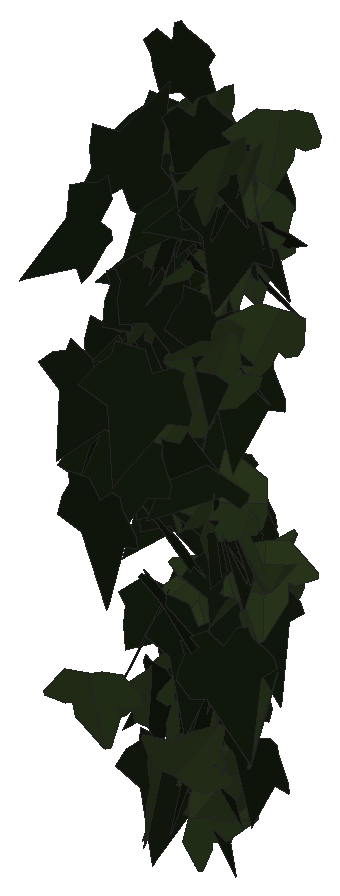
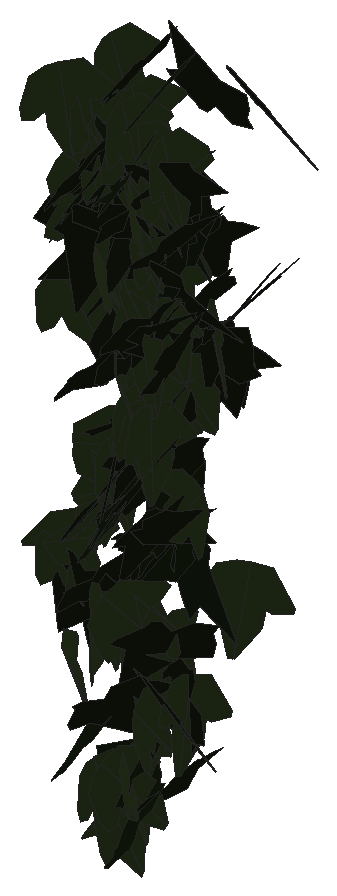
# SketchUp Ruby script. Lengths in inches.
U = 1.inch
M = Sketchup.active_model
def pt(a) = Geom::Point3d.new(a.map { |v| v * U })
def face(e, loops, mat)
  f = e.add_face(loops[0].map { |a| pt(a) })
  loops[1..].each { |l| e.add_face(l.map { |a| pt(a) }).erase! }
  f.material = f.back_material = mat if mat
  f
end
# faces: each face lists its corners as indices into pts; further lists are holes
def faces(e, pts, list, mat = nil) = list.each { |f| face(e, (f[0].is_a?(Array) ? f : [f]).map { |l| l.map { |i| pts[i] } }, mat) }
# xy, xz, yz: faces in a plane at the given z, y or x. An outline is a flat list of corners, or four numbers for a rectangle; further outlines are holes
def ring(l) = l.size == 4 ? [[l[0], l[1]], [l[2], l[1]], [l[2], l[3]], [l[0], l[3]]] : l.each_slice(2).to_a
def flat(e, list, mat, &to3) = list.each { |f| face(e, (f[0].is_a?(Array) ? f : [f]).map { |l| ring(l).map { |u, v| to3.(u, v) } }, mat) }
def xy(e, z, list, mat = nil) = flat(e, list, mat) { |x, y| [x, y, z] }
def xz(e, y, list, mat = nil) = flat(e, list, mat) { |x, z| [x, y, z] }
def yz(e, x, list, mat = nil) = flat(e, list, mat) { |y, z| [x, y, z] }
def lines(e, pts, list) = list.each { |a, b| e.add_line(pt(pts[a]), pt(pts[b])) }
# prism: a flat outline (further loops are holes) pulled along v
def prism(e, loops, v, mat = nil)
  f = face(e, loops, mat); d = Geom::Vector3d.new(v.map { |x| x * U })
  f.pushpull(f.normal.samedirection?(d) ? d.length : -d.length)
end
def box(e, o, s, mat = nil) = prism(e, [[o, [o[0] + s[0], o[1], o[2]], [o[0] + s[0], o[1] + s[1], o[2]], [o[0], o[1] + s[1], o[2]]]], [0, 0, s[2]], mat)
def at(x, y, z, deg = 0) = Geom::Transformation.translation(pt([x, y, z])) * Geom::Transformation.rotation(ORIGIN, Z_AXIS, deg.degrees)
def axes(o, x, y, z) = Geom::Transformation.new([*x, 0, *y, 0, *z, 0, *pt(o).to_a, 1])
def part(name) = M.definitions.add(name)
# library, detail: a bought-in or finely detailed component or shape, given as its bounding box
def library(name, o, s) = part(name).tap { |d| box(d.entities, o, s) }
def detail(e, o, s) = box(e.add_group.entities, o, s)
def put(e, d, t, mat = nil) = e.add_instance(d, t).tap { |i| i.material = mat if mat }
def group(e, t, mat = nil) = e.add_group.tap { |g| g.transformation = t; g.material = mat if mat }.entities
root = M.entities
M.materials.add("efeu1").color = [18, 25, 13]
M.materials.add("efeu2").color = [43, 57, 29]
c1 = part("ivyleaf_10")
p = [[0,0.5,-0.03],[-0.0625,2.02,-0.43],[-0.19,2.01,-0.46],[-0.54,1.05,-0.29],[-0.52,0.625,-0.18],[-0.83,0.76,-0.28],
  [-1.16,0.64,-0.33],[-1.15,0.33,-0.24],[-0.77,-0.39,0.02],[-0.3,-0.51,0.16],[0.04,-0.48,0.23],[-0.02,2.01,-0.4375],
  [-0.06,2.01,-0.43],[0.04,-0.49,0.23],[0.67,-0.49,0.14],[1.38,0.36,-0.2],[1.375,0.51,-0.24],[0.81,0.65,-0.19],
  [0.62,0.59,-0.15],[0.6,1.09,-0.28],[0.5,1.23,-0.31]]
faces(c1.entities,p,[[0,1,2,3,4,5,6,7,8,9,10],[11,12,0,13,14,15,16,17,18,19,20]],"efeu2")
c2 = part("ivyleaf_9")
p = [[1.54,2.16,1.25],[1.36,2.04,1.19],[-0.21,0.99,0.68],[-0.71,1.11,0.82],[-0.85,0.86,0.67],[-0.8,0.17,0.21],
  [-0.9,-0.01,0.1],[-0.67,-0.16,-0.02],[-0.08,-0.08,-0.05],[-0.03,-0.6,-0.4],[0.65,-0.88,-0.66],[0.83,-0.6,-0.49],
  [1.29,-0.42,-0.43],[1.8125,-0.07,-0.26],[1.21,0.44,0.15]]
faces(c2.entities,p,[[0,1,2,3,4,5,6,7,8,9,10,11,12,13,14]],"efeu1")
put(root,c1,axes([18.49,222.43,229.99],[0.23002,-0.33057,-0.29633],[-0.15826,0.25076,-0.40258],[0.41478,0.279,0.01073]))
put(root,c1,axes([18.22,223.25,227.8],[-0.37574,0.15973,-0.28863],[0.24252,-0.1628,-0.40581],[-0.22361,-0.44495,0.04487]))
put(root,c1,axes([18.43,222.98,224.79],[-0.0906,-0.46509,-0.15963],[0.04334,0.15413,-0.47367],[0.48981,-0.09967,0.01238]))
put(root,c2,axes([18.42,223.59,229.8],[-0.11921,-0.27208,0.4022],[-0.12254,-0.38388,-0.29601],[0.46986,-0.16914,0.02485]))
put(root,c1,axes([18.51,223.32,232.72],[0.01604,-0.49871,0.03217],[0.00614,-0.03199,-0.49894],[0.4997,0.0164,0.0051]))
put(root,c2,axes([18.41,223.64,231.55],[-0.15985,-0.43972,0.17633],[-0.02074,-0.17942,-0.46624],[0.47331,-0.15637,0.03912]))
put(root,c2,axes([18.82,223.33,230.9],[-0.44717,0.10536,0.19733],[-0.19143,0.04795,-0.45941],[-0.11573,-0.48641,-0.00254]))
put(root,c2,axes([18.55,223.72,227.49],[-0.316,-0.3588,0.14632],[-0.04704,-0.1519,-0.47404],[0.38462,-0.31335,0.06225]))
put(root,c2,axes([18.72,223.49,225.0625],[-0.4789,0.12444,-0.0719],[0.07015,-0.01592,-0.4948],[-0.12544,-0.484,-0.00221]))
put(root,c2,axes([18.56,223.48,232.52],[-0.39863,-0.28258,-0.10604],[0.08305,0.06619,-0.48859],[0.29017,-0.40715,-0.00584]))
put(root,c1,axes([18.67,223.45,228.82],[-0.0673,-0.49025,-0.07159],[0.02179,0.06925,-0.4947],[0.49497,-0.0697,0.01205]))
put(root,c1,axes([18.71,223.16,232.33],[-0.07169,-0.46603,0.16637],[-0.02755,-0.16409,-0.4715],[0.49407,-0.07677,-0.00215]))
put(root,c2,axes([18.45,222.9,230.46],[0.08987,-0.48242,-0.09591],[-0.01598,0.09459,-0.49071],[0.4916,0.09126,0.00159]))
put(root,c2,axes([18.42,223.4,225.875],[0.00253,-0.37791,-0.32737],[0.11638,0.31883,-0.36715],[0.48626,-0.07435,0.08958]))
put(root,c2,axes([18.44,222.44,229.3125],[-0.24213,0.0676,0.43221],[0.40007,-0.16562,0.25003],[0.17697,0.4669,0.02611]))
put(root,c2,axes([18.86,223.4,229.93],[-0.33647,-0.18993,0.31735],[-0.2156,-0.24787,-0.37693],[0.30051,-0.39049,0.08491]))
put(root,c1,axes([18.72,222.76,229.12],[-0.09175,-0.40686,0.27576],[0.04283,-0.28607,-0.40783],[0.48964,-0.05122,0.08734]))
put(root,c1,axes([19,223.41,230.66],[0.24717,0.01492,-0.43438],[-0.43424,-0.01272,-0.24753],[-0.01844,0.49962,0.00667]))
put(root,c1,axes([18.77,223.36,231.46],[0.0213,-0.48092,0.13513],[-0.01137,-0.13569,-0.4811],[0.49942,0.01742,-0.01671]))
put(root,c2,axes([18.54,223.41,227.57],[0.11099,-0.41936,-0.24864],[-0.03846,0.24667,-0.43321],[0.48601,0.11529,0.0225]))
put(root,c1,axes([18.71,223.19,230.1],[0.00725,-0.44774,0.22243],[0.07343,-0.21909,-0.44341],[0.49453,0.0391,0.06258]))
put(root,c2,axes([18.82,221.67,229.08],[-0.02563,0.08745,-0.49162],[-0.30019,0.39069,0.08515],[0.39904,0.29952,0.03248]))
put(root,c2,axes([18.52,223.41,233.75],[0.28205,-0.39313,-0.12607],[-0.02753,0.13444,-0.4808],[0.41194,0.27816,0.05419]))
put(root,c1,axes([18.81,222.95,231.91],[0.01487,-0.49894,-0.02902],[-0.00396,0.02891,-0.49915],[0.49976,0.01507,-0.00309]))
put(root,c2,axes([18.625,223.22,223.5],[-0.06473,-0.47171,0.15265],[0.02959,-0.15735,-0.47367],[0.49491,-0.05229,0.04829]))
put(root,c1,axes([18.76,222.76,231.3],[0.11483,-0.39119,-0.28946],[0.0705,0.30764,-0.3878],[0.4815,0.04824,0.12581]))
put(root,c2,axes([18.42,223.23,231.15],[0.14483,-0.22385,0.42298],[0.26952,-0.32703,-0.26535],[0.39545,0.30487,0.02593]))
put(root,c2,axes([18.68,221.58,229.74],[-0.11819,-0.39915,0.27696],[0.02609,-0.28984,-0.40658],[0.48513,-0.08165,0.08934]))
put(root,c2,axes([18.4,223.13,231.45],[0.17859,-0.27091,0.38041],[0.314,-0.23182,-0.31251],[0.3457,0.35052,0.08733]))
put(root,c1,axes([18.72,223.54,224.57],[0.11366,-0.35039,0.3381],[0.15787,-0.30191,-0.36596],[0.46061,0.18994,0.042]))
put(root,c1,axes([18.86,221.34,225.57],[-0.46112,-0.19068,-0.03179],[0.0291,0.01282,-0.49899],[0.19111,-0.46203,-0.00073]))
put(root,c1,axes([19.03,223.7,226.125],[-0.19329,-0.28552,0.36211],[-0.16913,-0.32138,-0.34368],[0.429,-0.25534,0.02766]))
put(root,c1,axes([18.7,222.99,230.05],[-0.40483,0.16773,-0.24078],[0.20233,-0.13761,-0.43604],[-0.21254,-0.45048,0.04355]))
put(root,c2,axes([18.71,223.46,230.34],[-0.05512,-0.47784,-0.1365],[0.0033,0.13698,-0.48086],[0.49694,-0.05391,-0.01195]))
put(root,c2,axes([18.47,222.98,224.71],[0.0622,-0.02561,-0.49545],[0.48938,0.08517,0.05704],[0.08147,-0.49203,0.03566]))
put(root,c2,axes([18.66,223.59,228.18],[0.18627,-0.46146,-0.04853],[-0.01392,0.04671,-0.49762],[0.4638,0.18673,0.00455]))
put(root,c1,axes([19.11,223.12,229.8125],[-0.42756,0.04442,0.25538],[-0.25395,0.02698,-0.42986],[-0.05197,-0.49729,-0.00051]))
put(root,c1,axes([18.93,223.43,232],[0.17479,-0.46471,-0.05906],[-0.01428,0.05773,-0.49645],[0.46824,0.17524,0.00691]))
put(root,c1,axes([18.96,222.5,230.7],[0.07805,-0.4605,-0.17847],[-0.01785,0.17794,-0.46693],[0.49355,0.07925,0.01134]))
put(root,c1,axes([18.97,223.13,228.67],[-0.21243,-0.4516,-0.03047],[0.00717,0.0303,-0.49903],[0.45257,-0.21246,-0.00639]))
put(root,c2,axes([19.03,222.75,231.67],[-0.39202,0.19463,-0.24175],[0.21966,-0.10113,-0.43763],[-0.21925,-0.44932,-0.00621]))
put(root,c1,axes([19,223.33,232.72],[-0.23758,-0.43928,0.02424],[-0.00273,-0.02608,-0.49931],[0.43994,-0.23738,0.00999]))
put(root,c2,axes([19.22,220.96,232.51],[-0.4655,0.1808,0.0249],[-0.02444,0.00584,-0.49937],[-0.18086,-0.46613,0.00341]))
put(root,c2,axes([18.87,223.66,231.97],[-0.11651,-0.46381,0.14595],[-0.0226,-0.14475,-0.47805],[0.48571,-0.118,0.01277]))
put(root,c1,axes([19.09,223.67,223.67],[-0.09524,-0.37066,0.32177],[-0.09347,-0.30808,-0.38256],[0.48187,-0.13302,-0.01061]))
put(root,c1,axes([19.03,223.07,230.37],[0.24768,-0.41489,-0.12854],[-0.04106,0.12494,-0.48239],[0.4324,0.24951,0.02782]))
put(root,c1,axes([19.01,223.45,223.72],[0.15733,-0.4744,0.01374],[0.00443,-0.01301,-0.49981],[0.47458,0.15739,0.00011]))
put(root,c2,axes([19.07,223.08,232.2],[-0.31124,-0.35892,0.15592],[-0.04886,-0.16203,-0.47049],[0.38826,-0.3081,0.06579]))
put(root,c1,axes([18.79,223.43,225.97],[0.4352,0.07159,0.23553],[0.23055,0.04915,-0.44094],[-0.08629,0.4924,0.00977]))
put(root,c1,axes([19.09,223.42,233.07],[-0.02939,-0.49624,0.05371],[0.01107,-0.05443,-0.4969],[0.49901,-0.02802,0.01418]))
put(root,c1,axes([19.07,223.36,228.85],[0.01693,-0.4832,0.12739],[0.03041,-0.12623,-0.48285],[0.49879,0.02409,0.02511]))
put(root,c1,axes([19.08,223.22,230.73],[0.04276,-0.41979,0.26823],[0.02782,-0.26678,-0.42196],[0.49739,0.05101,0.00054]))
put(root,c2,axes([19.15,222.14,226.1875],[-0.32069,0.26618,-0.27623],[0.21379,-0.17493,-0.41677],[-0.31851,-0.38542,-0.00162]))
put(root,c2,axes([18.76,223.64,223.13],[0.22105,-0.39181,0.21821],[0.10401,-0.19186,-0.44986],[0.43625,0.24428,-0.00332]))
put(root,c2,axes([19.01,221.78,232.66],[-0.35569,0.20594,0.28473],[0.24474,-0.14554,0.411],[0.25216,0.43175,0.00273]))
put(root,c2,axes([18.79,222.91,227.1],[0.02735,-0.29699,0.40131],[0.24681,-0.34132,-0.26942],[0.43398,0.21283,0.12793]))
put(root,c1,axes([19.15,223.62,223.13],[0.03474,-0.46755,0.17377],[0.01106,-0.17342,-0.46883],[0.49867,0.03641,-0.00171]))
put(root,c2,axes([18.95,222.94,228.15],[-0.00928,-0.34731,-0.35957],[0.02564,0.35883,-0.34725],[0.49926,-0.02488,0.01115]))
put(root,c1,axes([19.09,223.02,224.97],[0.06128,-0.43269,0.24295],[0.1161,-0.2255,-0.43089],[0.48246,0.10922,0.07283]))
put(root,c2,axes([18.95,222.45,231.02],[0.14227,-0.44698,-0.1731],[-0.02881,0.17227,-0.4685],[0.47846,0.14329,0.02326]))
put(root,c1,axes([19.08,223.31,230.34],[-0.11055,-0.33535,0.354],[0.16948,-0.36678,-0.29453],[0.45723,0.05487,0.19476]))
put(root,c2,axes([19.16,223.75,224.8125],[-0.23283,-0.44165,0.02713],[-0.00804,-0.02643,-0.49924],[0.44241,-0.23291,0.0052]))
put(root,c1,axes([19.125,223.48,229.27],[0.33317,-0.31949,0.19216],[0.13828,-0.13343,-0.4616],[0.34623,0.36072,-0.00055]))
put(root,c2,axes([18.99,223.47,232.49],[0.2856,-0.4104,0.00221],[0.00128,-0.0018,-0.5],[0.4104,0.28561,0.00002]))
put(root,c1,axes([19.3,222.95,233.03],[-0.08013,-0.47509,0.13368],[0.00933,-0.13686,-0.48081],[0.49345,-0.07456,0.0308]))
put(root,c2,axes([19.09,223.04,228.64],[-0.14371,-0.3551,0.32133],[0.12506,-0.35167,-0.3327],[0.46229,-0.01525,0.18989]))
put(root,c2,axes([19.24,221.5625,228.95],[-0.36621,-0.30924,-0.14235],[0.1108,0.08942,-0.4793],[0.32189,-0.38259,0.00304]))
put(root,c1,axes([19.36,222.6,229.26],[-0.17602,-0.37038,0.28607],[-0.04394,-0.29121,-0.40406],[0.46593,-0.16739,0.06996]))
put(root,c2,axes([19.38,223.59,231.69],[-0.45532,-0.19539,-0.06712],[0.06362,0.02194,-0.49545],[0.19656,-0.45972,0.00488]))
put(root,c2,axes([18.95,223.52,223.67],[0.17403,-0.35204,0.30948],[0.17894,-0.25523,-0.39095],[0.43324,0.24683,0.03716]))
put(root,c1,axes([19.36,222.94,229.84],[0.00912,-0.41573,0.27764],[0.05426,-0.27522,-0.41389],[0.49696,0.03768,0.04009]))
put(root,c2,axes([19.12,223.72,228.09],[0.14057,-0.16887,-0.44914],[0.40301,-0.21246,0.20602],[-0.26043,-0.41993,0.07638]))
put(root,c1,axes([19.34,223.56,231.03],[0.1772,-0.41935,0.20676],[0.0732,-0.1935,-0.45519],[0.46178,0.19159,-0.00718]))
put(root,c2,axes([19.1,222.69,226.16],[0.00637,-0.31139,0.39115],[0.22861,-0.34608,-0.27923],[0.44463,0.1824,0.13797]))
put(root,c2,axes([19.1,223.49,227.6],[0.2118,-0.42089,0.16732],[0.07928,-0.14741,-0.47115],[0.44593,0.22611,0.0043]))
put(root,c1,axes([19.3,222.93,223.15],[0.07077,-0.21703,-0.44485],[0.18626,0.42802,-0.17919],[0.45858,-0.14035,0.14143]))
put(root,c2,axes([19.21,223.76,227.27],[0.01542,-0.37526,0.33006],[0.05245,-0.32718,-0.37444],[0.497,0.04617,0.02927]))
put(root,c1,axes([19.51,223.46,223.44],[-0.02066,-0.4994,0.01327],[-0.00139,-0.01322,-0.49982],[0.49957,-0.02069,-0.00084]))
put(root,c1,axes([19.5,223.375,226.08],[0.08402,-0.49207,-0.02848],[-0.00769,0.02758,-0.49918],[0.49283,0.08432,-0.00293]))
put(root,c2,axes([19.5625,223.09,228.41],[-0.32859,-0.31081,0.21314],[-0.03881,-0.25337,-0.4293],[0.37487,-0.29867,0.14238]))
put(root,c2,axes([19.3,223.08,232.28],[0.21048,-0.41575,-0.18125],[-0.04013,0.18197,-0.46398],[0.45176,0.20987,0.04324]))
put(root,c2,axes([19.16,223.33,229.82],[0.25074,-0.27453,0.33431],[0.23382,-0.23909,-0.3717],[0.36395,0.34274,0.00849]))
put(root,c2,axes([19.41,223.56,227.34],[-0.09365,-0.41897,0.2563],[0.05854,-0.26858,-0.41766],[0.48765,-0.04822,0.09936]))
put(root,c1,axes([19.77,222.96,231.41],[0.33072,-0.13862,-0.34844],[-0.31426,0.15104,-0.35837],[0.20461,0.45604,0.01278]))
put(root,c2,axes([19.48,223.61,226.39],[-0.13623,-0.47148,0.09566],[-0.00391,-0.09834,-0.49022],[0.48107,-0.13431,0.02311]))
put(root,c1,axes([19.62,223.03,227.84],[0.01891,-0.49879,0.02917],[0.00353,-0.02906,-0.49914],[0.49963,0.01908,0.00243]))
put(root,c2,axes([19.35,223.69,227.63],[0.11155,-0.46219,0.15472],[0.04348,-0.14865,-0.47541],[0.48545,0.11952,0.00703]))
put(root,c2,axes([19.26,223.31,231.28],[0.45873,-0.16514,0.11087],[0.10779,-0.02783,-0.48745],[0.16717,0.47112,0.01007]))
put(root,c2,axes([19.79,223.24,231.94],[-0.24308,-0.16784,0.40341],[-0.28493,-0.28909,-0.29196],[0.33125,-0.37183,0.0449]))
put(root,c2,axes([19.55,222.7,224.7],[-0.29017,0.05517,-0.40343],[0.37193,-0.16574,-0.29018],[-0.16575,-0.46849,0.05515]))
put(root,c2,axes([19.49,222.63,226.01],[0.00471,-0.48333,0.12796],[-0.00653,-0.12802,-0.48329],[0.49994,0.00288,-0.00752]))
put(root,c2,axes([19.85,222.85,232.43],[-0.41021,0.2599,-0.11906],[0.0992,-0.06588,-0.48561],[-0.26811,-0.42203,0.00249]))
put(root,c2,axes([19.68,223.16,231.58],[0.31922,0.365,-0.12198],[-0.1147,-0.06104,-0.48282],[-0.36735,0.33623,0.04476]))
put(root,c1,axes([19.42,221.86,224.07],[0.0715,-0.07913,0.48849],[0.34442,-0.34644,-0.10653],[0.35533,0.35173,0.00497]))
put(root,c1,axes([19.46,223.61,225.26],[-0.24668,0.11526,0.41936],[0.35796,-0.22001,0.27103],[0.24701,0.43395,0.02603]))
put(root,c1,axes([19.98,223.01,227.87],[-0.0281,0.03727,0.49782],[-0.34659,-0.36031,0.00741],[0.35929,-0.34466,0.04608]))
put(root,c2,axes([19.54,223.53,229.4375],[-0.04975,-0.49165,0.07618],[0.02043,-0.07851,-0.49337],[0.4971,-0.04598,0.0279]))
put(root,c2,axes([19.53,223.5,227.49],[0.06551,-0.48323,0.11045],[0.00541,-0.11071,-0.48756],[0.49566,0.06507,-0.00928]))
put(root,c1,axes([19.77,223.09,232.1875],[-0.00424,-0.49081,0.09533],[0.00634,-0.09538,-0.49078],[0.49994,-0.00295,0.00703]))
put(root,c2,axes([19.72,221.4,230.27],[-0.24006,-0.4386,0.00023],[0.00133,-0.001,-0.5],[0.4386,-0.24006,0.00165]))
put(root,c1,axes([19.84,222.73,230.05],[-0.06726,-0.11811,-0.48117],[-0.18313,-0.44527,0.13489],[-0.46037,0.19438,0.01664]))
put(root,c1,axes([19.8,223.25,231.45],[-0.3758,-0.32622,-0.04852],[0.04268,0.02483,-0.49756],[0.32703,-0.37811,0.00918]))
put(root,c2,axes([19.59,222.88,230.39],[0.01086,-0.48734,0.11127],[0.01335,-0.11097,-0.48735],[0.4997,0.01356,0.0106]))
put(root,c2,axes([19.57,222.52,233.4],[0.23247,-0.41318,-0.15888],[-0.04017,0.15902,-0.47233],[0.44085,0.23237,0.04074]))
put(root,c2,axes([19.58,223.71,223.98],[0.03174,-0.42344,0.26399],[0.0731,-0.25773,-0.42218],[0.49361,0.0654,0.04555]))
put(root,c2,axes([19.64,223.71,232.32],[0.0226,-0.48238,0.12961],[-0.00606,-0.12999,-0.48277],[0.49945,0.02025,-0.01172]))
put(root,c2,axes([19.67,220.46,228.85],[0.08958,-0.47536,0.12654],[0.02994,-0.12312,-0.48368],[0.491,0.09423,0.00641]))
put(root,c2,axes([19.69,223.23,232.05],[0.2557,-0.3933,-0.173],[-0.07428,0.15783,-0.46859],[0.4232,0.26533,0.02228]))
put(root,c1,axes([19.61,223.37,232.14],[0.27678,-0.14604,0.38995],[0.38387,-0.09197,-0.3069],[0.16137,0.46927,0.06121]))
put(root,c1,axes([19.875,222.43,229.625],[-0.26661,-0.41632,0.07483],[0.04533,0.05982,0.49433],[-0.42056,0.27037,0.00584]))
put(root,c1,axes([20.04,223.26,232.04],[-0.2426,-0.29206,0.32534],[-0.04501,-0.35341,-0.35082],[0.43488,-0.19951,0.14518]))
put(root,c1,axes([19.68,223.125,227.41],[-0.24154,0.15113,-0.41088],[0.32697,-0.24978,-0.28409],[-0.29112,-0.40592,0.02183]))
put(root,c1,axes([20,222.99,232.76],[-0.02972,-0.497,0.04586],[-0.0048,-0.04565,-0.49789],[0.49909,-0.03003,-0.00206]))
put(root,c2,axes([19.77,223.46,226.3],[-0.24751,-0.16791,-0.40068],[0.34664,0.20165,-0.29863],[0.26188,-0.42561,0.01659]))
put(root,c1,axes([19.95,223.09,226.58],[0.06108,0.16228,-0.46897],[0.10556,0.45745,0.17204],[0.4849,-0.12003,0.02162]))
put(root,c1,axes([19.7,222.65,224.85],[0.09075,-0.03401,0.49052],[0.42915,-0.23799,-0.09589],[0.23999,0.43841,-0.01401]))
put(root,c1,axes([20.125,223.35,230.32],[-0.25427,-0.37056,0.21916],[-0.0515,-0.22652,-0.44276],[0.42743,-0.24774,0.07702]))
put(root,c1,axes([19.98,223.45,224.96],[0.32696,-0.35306,0.13582],[0.0796,-0.11129,-0.48091],[0.36981,0.3361,-0.01657]))
put(root,c2,axes([19.91,222.88,232],[-0.08275,-0.46424,0.16624],[0.04236,-0.17464,-0.46659],[0.49128,-0.06314,0.06824]))
put(root,c1,axes([19.88,221.88,224.5],[-0.3691,-0.23393,0.24299],[0.23229,0.08488,0.43455],[-0.24456,0.43367,0.04602]))
put(root,c1,axes([20.15,223.38,226.66],[-0.15839,-0.45075,0.14743],[-0.03909,-0.1425,-0.47767],[0.47264,-0.16284,0.00991]))
put(root,c2,axes([19.92,222.65,225.86],[0.00222,-0.45186,-0.21405],[-0.01356,0.21392,-0.45172],[0.49981,0.00781,-0.0113]))
put(root,c1,axes([20.05,223.29,226.91],[0.26233,0.42413,-0.03595],[-0.02188,-0.02874,-0.49869],[-0.42509,0.26322,0.00348]))
put(root,c1,axes([20.18,222.28,233.2],[-0.03785,-0.49578,0.05262],[-0.00793,-0.05217,-0.49721],[0.4985,-0.03847,-0.00391]))
put(root,c1,axes([20.23,223.36,233.22],[-0.32445,-0.37236,0.078],[-0.00958,-0.09449,-0.4909],[0.38032,-0.32004,0.05418]))
